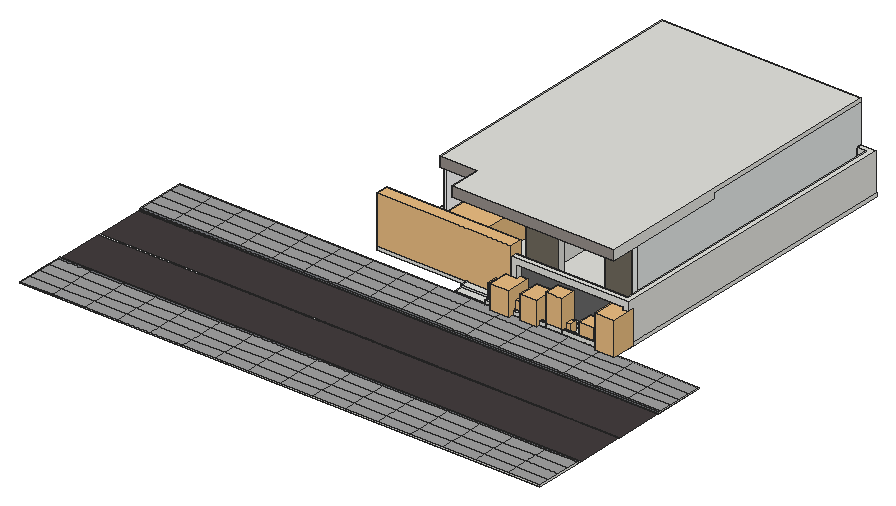
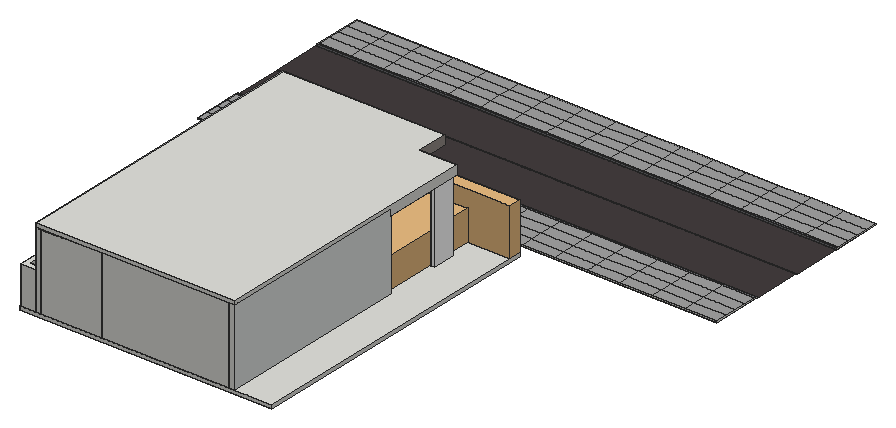
# SketchUp Ruby script. Lengths in inches.
U = 1.inch
M = Sketchup.active_model
def pt(a) = Geom::Point3d.new(a.map { |v| v * U })
def face(e, loops, mat)
  f = e.add_face(loops[0].map { |a| pt(a) })
  loops[1..].each { |l| e.add_face(l.map { |a| pt(a) }).erase! }
  f.material = f.back_material = mat if mat
  f
end
# faces: each face lists its corners as indices into pts; further lists are holes
def faces(e, pts, list, mat = nil) = list.each { |f| face(e, (f[0].is_a?(Array) ? f : [f]).map { |l| l.map { |i| pts[i] } }, mat) }
# xy, xz, yz: faces in a plane at the given z, y or x. An outline is a flat list of corners, or four numbers for a rectangle; further outlines are holes
def ring(l) = l.size == 4 ? [[l[0], l[1]], [l[2], l[1]], [l[2], l[3]], [l[0], l[3]]] : l.each_slice(2).to_a
def flat(e, list, mat, &to3) = list.each { |f| face(e, (f[0].is_a?(Array) ? f : [f]).map { |l| ring(l).map { |u, v| to3.(u, v) } }, mat) }
def xy(e, z, list, mat = nil) = flat(e, list, mat) { |x, y| [x, y, z] }
def xz(e, y, list, mat = nil) = flat(e, list, mat) { |x, z| [x, y, z] }
def yz(e, x, list, mat = nil) = flat(e, list, mat) { |y, z| [x, y, z] }
def lines(e, pts, list) = list.each { |a, b| e.add_line(pt(pts[a]), pt(pts[b])) }
# prism: a flat outline (further loops are holes) pulled along v
def prism(e, loops, v, mat = nil)
  f = face(e, loops, mat); d = Geom::Vector3d.new(v.map { |x| x * U })
  f.pushpull(f.normal.samedirection?(d) ? d.length : -d.length)
end
def box(e, o, s, mat = nil) = prism(e, [[o, [o[0] + s[0], o[1], o[2]], [o[0] + s[0], o[1] + s[1], o[2]], [o[0], o[1] + s[1], o[2]]]], [0, 0, s[2]], mat)
def at(x, y, z, deg = 0) = Geom::Transformation.translation(pt([x, y, z])) * Geom::Transformation.rotation(ORIGIN, Z_AXIS, deg.degrees)
def axes(o, x, y, z) = Geom::Transformation.new([*x, 0, *y, 0, *z, 0, *pt(o).to_a, 1])
def part(name) = M.definitions.add(name)
# library, detail: a bought-in or finely detailed component or shape, given as its bounding box
def library(name, o, s) = part(name).tap { |d| box(d.entities, o, s) }
def detail(e, o, s) = box(e.add_group.entities, o, s)
def put(e, d, t, mat = nil) = e.add_instance(d, t).tap { |i| i.material = mat if mat }
def group(e, t, mat = nil) = e.add_group.tap { |g| g.transformation = t; g.material = mat if mat }.entities
root = M.entities
M.materials.add("Kamosho - kamn7918 33.43cm").color = [255, 255, 255]
M.materials.add("Marble C 150cm").color = [150, 142, 138]
M.materials.add("Plain White Flat 3698829 28cm").color = [227, 230, 229]
M.materials.add("Roof Tiles A01 100cm\#1").color = [100, 100, 100]
M.materials.add("Stone C 250cm").color = [107, 104, 102]
M.materials.add("Stone G 100cm\#1").color = [112, 105, 93]
M.materials.add("[Asphalt_New]").color = [68, 61, 63]
M.materials.add("[Color_001]").color = [226, 226, 226]
M.materials.add("[Stone_Pavers_Flagstone_Gray]").color = [162, 162, 162]
M.materials.add("[Stone_Pavers_Walk]").color = [113, 115, 119]
c1 = library("Car 038",[-41.0625,-100.42,-1.26],[82.125,200.85,59.95])
c2 = library("Gate 243 015",[-82.73,-9.65,0],[165.46,19.3,75.06])
c3 = part("Roads11")
xy(c3.entities,0,[[0,0,78.74,393.7],[236.22,0,314.96,393.7]])
xy(c3.entities,0,[[80.71,0,156.3,393.7],[158.66,0,234.25,393.7]],"[Asphalt_New]")
xy(c3.entities,0,[[78.74,0,80.71,393.7],[156.3,0,158.66,393.7],[234.25,0,236.22,393.7]],"[Color_001]")
xy(c3.entities,1.97,[[0,0,18.7,24.61],[18.7,0,37.4,24.61],[37.4,0,56.1,24.61],[56.1,0,74.8,24.61],[240.16,0,258.86,24.61],
  [258.86,0,277.56,24.61],[277.56,0,296.26,24.61],[296.26,0,314.96,24.61],[0,24.61,18.7,49.21],[18.7,24.61,37.4,49.21],
  [37.4,24.61,56.1,49.21],[56.1,24.61,74.8,49.21],[240.16,24.61,258.86,49.21],[258.86,24.61,277.56,49.21],[277.56,24.61,296.26,49.21],
  [296.26,24.61,314.96,49.21],[0,49.21,18.7,73.82],[18.7,49.21,37.4,73.82],[37.4,49.21,56.1,73.82],[56.1,49.21,74.8,73.82],
  [240.16,49.21,258.86,73.82],[258.86,49.21,277.56,73.82],[277.56,49.21,296.26,73.82],[296.26,49.21,314.96,73.82],[0,73.82,18.7,98.43],
  [18.7,73.82,37.4,98.43],[37.4,73.82,56.1,98.43],[56.1,73.82,74.8,98.43],[240.16,73.82,258.86,98.43],[258.86,73.82,277.56,98.43],
  [277.56,73.82,296.26,98.43],[296.26,73.82,314.96,98.43],[0,98.43,18.7,123.03],[18.7,98.43,37.4,123.03],[37.4,98.43,56.1,123.03],
  [56.1,98.43,74.8,123.03],[240.16,98.43,258.86,123.03],[258.86,98.43,277.56,123.03],[277.56,98.43,296.26,123.03],[296.26,98.43,314.96,123.03],
  [0,123.03,18.7,147.64],[18.7,123.03,37.4,147.64],[37.4,123.03,56.1,147.64],[56.1,123.03,74.8,147.64],[240.16,123.03,258.86,147.64],
  [258.86,123.03,277.56,147.64],[277.56,123.03,296.26,147.64],[296.26,123.03,314.96,147.64],[0,147.64,18.7,172.24],[18.7,147.64,37.4,172.24],
  [37.4,147.64,56.1,172.24],[56.1,147.64,74.8,172.24],[240.16,147.64,258.86,172.24],[258.86,147.64,277.56,172.24],[277.56,147.64,296.26,172.24],
  [296.26,147.64,314.96,172.24],[0,172.24,18.7,196.85],[18.7,172.24,37.4,196.85],[37.4,172.24,56.1,196.85],[56.1,172.24,74.8,196.85],
  [240.16,172.24,258.86,196.85],[258.86,172.24,277.56,196.85],[277.56,172.24,296.26,196.85],[296.26,172.24,314.96,196.85],[0,196.85,18.7,221.46],
  [18.7,196.85,37.4,221.46],[37.4,196.85,56.1,221.46],[56.1,196.85,74.8,221.46],[240.16,196.85,258.86,221.46],[258.86,196.85,277.56,221.46],
  [277.56,196.85,296.26,221.46],[296.26,196.85,314.96,221.46],[0,221.46,18.7,246.0625],[18.7,221.46,37.4,246.0625],[37.4,221.46,56.1,246.0625],
  [56.1,221.46,74.8,246.0625],[240.16,221.46,258.86,246.0625],[258.86,221.46,277.56,246.0625],[277.56,221.46,296.26,246.0625],[296.26,221.46,314.96,246.0625],
  [0,246.0625,18.7,270.67],[18.7,246.0625,37.4,270.67],[37.4,246.0625,56.1,270.67],[56.1,246.0625,74.8,270.67],[240.16,246.0625,258.86,270.67],
  [258.86,246.0625,277.56,270.67],[277.56,246.0625,296.26,270.67],[296.26,246.0625,314.96,270.67],[0,270.67,18.7,295.28],[18.7,270.67,37.4,295.28],
  [37.4,270.67,56.1,295.28],[56.1,270.67,74.8,295.28],[240.16,270.67,258.86,295.28],[258.86,270.67,277.56,295.28],[277.56,270.67,296.26,295.28],
  [296.26,270.67,314.96,295.28],[0,295.28,18.7,319.88],[18.7,295.28,37.4,319.88],[37.4,295.28,56.1,319.88],[56.1,295.28,74.8,319.88],
  [240.16,295.28,258.86,319.88],[258.86,295.28,277.56,319.88],[277.56,295.28,296.26,319.88],[296.26,295.28,314.96,319.88],[0,319.88,18.7,344.49],
  [18.7,319.88,37.4,344.49],[37.4,319.88,56.1,344.49],[56.1,319.88,74.8,344.49],[240.16,319.88,258.86,344.49],[258.86,319.88,277.56,344.49],
  [277.56,319.88,296.26,344.49],[296.26,319.88,314.96,344.49],[0,344.49,18.7,369.09],[18.7,344.49,37.4,369.09],[37.4,344.49,56.1,369.09],
  [56.1,344.49,74.8,369.09],[240.16,344.49,258.86,369.09],[258.86,344.49,277.56,369.09],[277.56,344.49,296.26,369.09],[296.26,344.49,314.96,369.09],
  [0,369.09,18.7,393.7],[18.7,369.09,37.4,393.7],[37.4,369.09,56.1,393.7],[56.1,369.09,74.8,393.7],[240.16,369.09,258.86,393.7],
  [258.86,369.09,277.56,393.7],[277.56,369.09,296.26,393.7],[296.26,369.09,314.96,393.7]],"[Stone_Pavers_Flagstone_Gray]")
xy(c3.entities,1.97,[[74.8,0,78.74,393.7],[236.22,0,240.16,393.7]],"[Stone_Pavers_Walk]")
xz(c3.entities,0,[[0,0,74.8,1.97],[74.8,0,78.74,1.97],[236.22,0,240.16,1.97],[240.16,0,314.96,1.97]])
xz(c3.entities,393.7,[[0,0,74.8,1.97],[74.8,0,78.74,1.97],[236.22,0,240.16,1.97],[240.16,0,314.96,1.97]])
yz(c3.entities,0,[[0,0,393.7,1.97]])
yz(c3.entities,78.74,[[0,0,393.7,1.97]],"[Stone_Pavers_Walk]")
yz(c3.entities,236.22,[[0,0,393.7,1.97]],"[Stone_Pavers_Walk]")
yz(c3.entities,314.96,[[0,0,393.7,1.97]])
c4 = library("Door 243 065",[-19.36,-2.49,0],[38.72,4.98,81.96])
c5 = library("Fouquieria splendens 002",[-30.26,-26.69,-2.27],[57.52,65.08,116.59])
c6 = part("Group\#8")
box(c6.entities,[0,0,0],[96,4.5,120])
c7 = part("Group\#4")
box(c7.entities,[0,0,0],[201,9,120])
c8 = part("Group\#7")
prism(c8.entities,[[[6,4.5,0],[0,4.5,0],[0,4.5,120],[96,4.5,120],[96,4.5,0],[36,4.5,0],[36,4.5,84],[6,4.5,84]]],[0,-4.5,0])
c9 = part("Group\#9")
box(c9.entities,[0,0,0],[96,4.5,120])
c10 = part("Group\#6")
xy(c10.entities,0,[[0,0,90,4.5],[126,0,126,4.5,132,4.5,132,148.5,136.5,148.5,136.5,64.5,160.5,64.5,160.5,60,136.5,60,136.5,0],[190.5,60,190.5,64.5,196.5,64.5,196.5,148.5,201,148.5,201,60]])
xy(c10.entities,84,[[90,0,126,4.5],[160.5,60,190.5,64.5]])
xy(c10.entities,120,[[0,0,136.5,0,136.5,60,201,60,201,148.5,196.5,148.5,196.5,64.5,136.5,64.5,136.5,148.5,132,148.5,132,4.5,0,4.5]])
xz(c10.entities,0,[[0,0,90,0,90,84,126,84,126,0,136.5,0,136.5,120,0,120]])
xz(c10.entities,4.5,[[0,0,0,120,132,120,132,0,126,0,126,84,90,84,90,0]])
xz(c10.entities,60,[[136.5,0,160.5,0,160.5,84,190.5,84,190.5,0,201,0,201,120,136.5,120]])
xz(c10.entities,64.5,[[136.5,0,136.5,120,196.5,120,196.5,0,190.5,0,190.5,84,160.5,84,160.5,0]])
xz(c10.entities,148.5,[[132,0,136.5,120],[196.5,0,201,120]])
yz(c10.entities,0,[[0,0,4.5,120]])
yz(c10.entities,90,[[0,0,4.5,84]])
yz(c10.entities,126,[[0,0,4.5,84]])
yz(c10.entities,132,[[4.5,0,148.5,120]])
yz(c10.entities,136.5,[[0,0,60,120],[64.5,0,148.5,120]])
yz(c10.entities,160.5,[[60,0,64.5,84]])
yz(c10.entities,190.5,[[60,0,64.5,84]])
yz(c10.entities,196.5,[[64.5,0,148.5,120]])
yz(c10.entities,201,[[60,0,148.5,120]])
c11 = library("Potted Plant 02",[-16.98,-19.78,0],[30.04,38.68,37.52])
c12 = library("Sedum Plant 66-24",[-7.97,-7.95,0.04],[16.42,16.31,19.57])
c13 = library("Potted Plant 08",[-13.67,-16.93,0],[26.14,33.37,37.04])
c14 = library("Potted Plant 50-12",[-6.11,-5.26,0],[11.24,10.56,13.41])
c15 = library("Indoor Plant 004",[-26.75,-21.09,0],[44.44,41.03,87.36])
c16 = library("Large Boxwood Plant 66-28",[-21.37,-20.87,0.32],[41.28,41.36,41.23])
xy(root,-0.6875,[[771.74,314.96,976.61,339.27]])
xy(root,0.72,[[775.24,318.46,973.11,339.27]])
xy(root,6,[[792.9,339.27,970.5,348.27],[640.5,396.46,645.56,433.84]])
xy(root,7.72,[[771.74,314.96,976.61,314.96,976.61,339.27,973.11,339.27,973.11,318.46,775.24,318.46,775.24,339.27,771.74,339.27]])
xy(root,116.875,[[698.8,339.27,955.5,538.46],[640.5,389.4,640.5,396.46,645.56,396.46,645.56,433.84,640.5,433.84,640.5,519.27,698.8,519.27,698.8,389.4],[640.5,396.46,645.56,433.84]])
xy(root,126,[[640.5,519.27,640.5,829.77,955.5,829.77,955.5,538.46,698.8,538.46,698.8,519.27]])
xy(root,132,[[698.8,339.27,955.5,339.27,955.5,829.77,640.5,829.77,640.5,389.4,698.8,389.4]])
xz(root,314.96,[[771.74,-0.6875,976.61,7.72]])
xz(root,318.46,[[775.24,0.72,973.11,7.72]])
xz(root,339.27,[[771.74,-0.6875,771.74,7.72,775.24,7.72,775.24,0.72,973.11,0.72,973.11,7.72,976.61,7.72,976.61,-0.6875]])
xz(root,339.27,[[698.8,116.875,955.5,132]],"Marble C 150cm")
xz(root,389.4,[[640.5,116.875,698.8,132]],"Marble C 150cm")
xz(root,396.46,[[640.5,6,645.56,116.875]],"Kamosho - kamn7918 33.43cm")
xz(root,433.84,[[640.5,6,645.56,116.875]],"Kamosho - kamn7918 33.43cm")
xz(root,519.27,[[640.5,116.875,698.8,126]])
xz(root,538.46,[[698.8,116.875,955.5,126]])
xz(root,829.77,[[640.5,126,955.5,132]])
yz(root,640.5,[[389.4,116.875,389.4,132,829.77,132,829.77,126,519.27,126,519.27,116.875]])
yz(root,640.5,[[396.46,6,433.84,116.875]],"Kamosho - kamn7918 33.43cm")
yz(root,645.56,[[396.46,6,433.84,116.875]],"Kamosho - kamn7918 33.43cm")
yz(root,698.8,[[519.27,116.875,538.46,126]])
yz(root,698.8,[[339.27,116.875,389.4,132]],"Marble C 150cm")
yz(root,771.74,[[314.96,-0.6875,339.27,7.72]])
yz(root,775.24,[[318.46,0.72,339.27,7.72]])
yz(root,955.5,[[339.27,116.875,538.46,116.875,538.46,126,829.77,126,829.77,132,339.27,132]])
yz(root,973.11,[[318.46,0.72,339.27,7.72]])
yz(root,976.61,[[314.96,-0.6875,339.27,7.72]])
put(root,c1,axes([680.67,428.24,7.01],[-0.8,0,0],[0,-0.8,0],[0,0,0.8]))
g1 = group(root,at(649.33,519.17,6),"Stone C 250cm")
xy(g1,0,[[0,0,74.67,0.1]])
xy(g1,110.5625,[[0,0,74.67,0.1]])
xz(g1,0,[[0,0,74.67,110.5625]],"Stone G 100cm\#1")
xz(g1,0.1,[[0,0,74.67,110.5625]],"Stone C 250cm")
yz(g1,0,[[0,0,0.1,110.5625]],"Stone C 250cm")
yz(g1,74.67,[[0,0,0.1,110.5625]],"Stone C 250cm")
put(root,c2,axes([686.72,348.85,5.96],[1.28393,0,0],[0,1,0],[0,0,1]))
put(root,c3,axes([287.48,314.96,-0.6875],[0,-1,0],[2.0904,0,0],[0,0,1]))
g2 = group(root,at(723.74,315.27,-0.6875))
prism(g2,[[[48,0,0],[48,24,0],[48,24,6.6875],[48,12,6.6875],[48,12,3.375],[48,0,3.375]]],[-48,0,0])
put(root,c4,axes([754.5,529.84,6],[0.92977,0,0],[0,-0.44,0],[0,0,1.02]))
put(root,c5,axes([780.33,325.91,1.28],[0.2484,0,0],[0,0.2484,0],[0,0,0.2484]))
g3 = group(root,at(640.5,333.91,0))
box(g3,[-60,5.37,0],[399,490.5,6])
g4 = group(root,at(640.5,339.27,6))
put(g4,c6,at(210,486,0))
put(g4,c7,at(9,481.5,0))
g5 = group(g4,at(306,0,0))
xy(g5,0,[[0,48,9,490.5]])
xy(g5,120,[[0,48,9,490.5]])
xz(g5,48,[[0,0,9,120]],"Plain White Flat 3698829 28cm")
xz(g5,490.5,[[0,0,9,120]])
yz(g5,0,[[48,0,490.5,120]])
yz(g5,9,[[48,0,490.5,120]],"Plain White Flat 3698829 28cm")
put(g4,c8,at(210,433.5,0))
g6 = group(g4,at(0,0,0))
xy(g6,0,[[0,180,9,490.5]])
xy(g6,120,[[0,180,9,490.5]])
xz(g6,180,[[0,0,9,120]])
xz(g6,490.5,[[0,0,9,120]])
yz(g6,0,[[180,0,490.5,120]],"Plain White Flat 3698829 28cm")
yz(g6,9,[[180,0,490.5,120]])
put(g4,c9,at(210,225,0))
g7 = group(g4,at(9,48,0))
xy(g7,0,[[129,0,129,132,123,132,123,141,138,141,138,9,297,9,297,0],[0,132,87,141]])
xy(g7,24,[[181.5,0,253.5,9]])
xy(g7,84,[[87,132,123,141]])
xy(g7,87,[[181.5,0,217.5,9],[217.5,0,253.5,9]])
xy(g7,120,[[129,0,297,0,297,9,138,9,138,141,0,141,0,132,129,132]])
xz(g7,0,[[[129,0,297,120],[181.5,24,253.5,87]]],"Stone G 100cm\#1")
xz(g7,9,[[[138,0,297,120],[181.5,24,253.5,87]]])
xz(g7,132,[[0,0,87,0,87,84,123,84,123,0,129,0,129,120,0,120]],"Kamosho - kamn7918 33.43cm")
xz(g7,141,[[0,0,0,120,138,120,138,0,123,0,123,84,87,84,87,0]])
yz(g7,0,[[132,0,141,120]])
yz(g7,87,[[132,0,141,84]])
yz(g7,123,[[132,0,141,84]])
yz(g7,129,[[0,0,132,120]],"Kamosho - kamn7918 33.43cm")
yz(g7,138,[[9,0,141,120]])
yz(g7,181.5,[[0,24,9,87]])
yz(g7,253.5,[[0,24,9,87]])
yz(g7,297,[[0,0,9,120]])
put(g4,c10,at(9,333,0))
put(root,c11,at(801.89,327.1,0.72))
put(root,c12,at(819.21,328.36,0.72))
put(root,c13,at(844.02,327.31,0.72))
put(root,c14,at(865.11,331.51,0.72))
put(root,c15,axes([882.78,327.71,0.72],[0.58,0,0],[0,0.58,0],[0,0,0.58]))
g8 = group(root,at(955.5,339.27,6))
xy(g8,0,[[-162.6,0,-162.6,9,15,9,15,481.5,0,481.5,0,490.5,24,490.5,24,0,15,0,15,8,-153.11,8,-153.11,0]])
xy(g8,50.75,[[-153.35,0,14.75,8]])
xy(g8,60,[[-162.6,0,24,0,24,490.5,0,490.5,0,481.5,15,481.5,15,9,-162.6,9]])
xz(g8,0,[[-162.6,0,-153.11,0,-153.35,50.75,14.75,50.75,15,0,24,0,24,60,-162.6,60]])
xz(g8,8,[[-153.11,0,15,0,14.75,50.75,-153.35,50.75]],"Roof Tiles A01 100cm\#1")
xz(g8,9,[[-162.6,0,15,60]])
xz(g8,481.5,[[0,0,15,60]])
xz(g8,490.5,[[0,0,24,60]])
yz(g8,-162.6,[[0,0,9,60]])
yz(g8,0,[[481.5,0,490.5,60]])
yz(g8,15,[[9,0,481.5,60]])
yz(g8,24,[[0,0,490.5,60]])
p = [[-153.35,0,50.75],[-153.11,0,0],[-153.11,8,0],[-153.35,8,50.75],[15,0,0],[14.75,0,50.75],
  [14.75,8,50.75],[15,8,0]]
faces(g8,p,[[0,1,2,3],[4,5,6,7]])
put(root,c14,at(895.5625,328.58,0.72))
put(root,c16,axes([929.33,330.77,0.13],[0.59,0,0],[0,0.59,0],[0,0,0.59]))
put(root,c12,at(952.39,328.36,0.72))
put(root,c11,axes([966.49,329.47,0.72],[1,0,0],[0,1,0],[0,0,1.39]))
